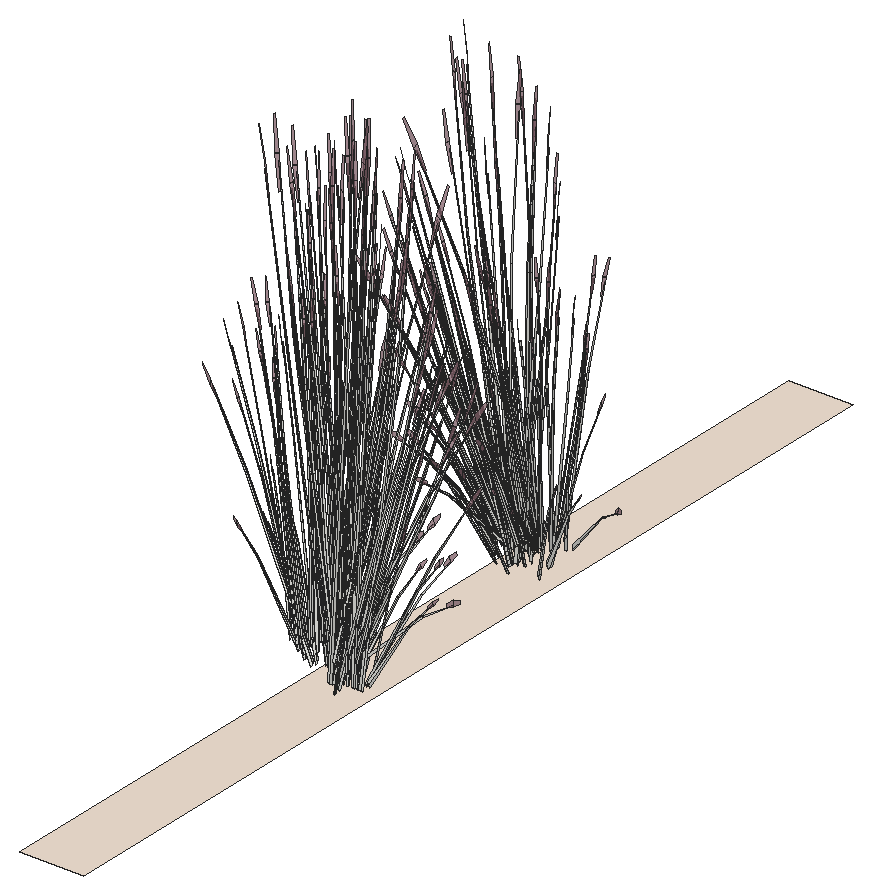
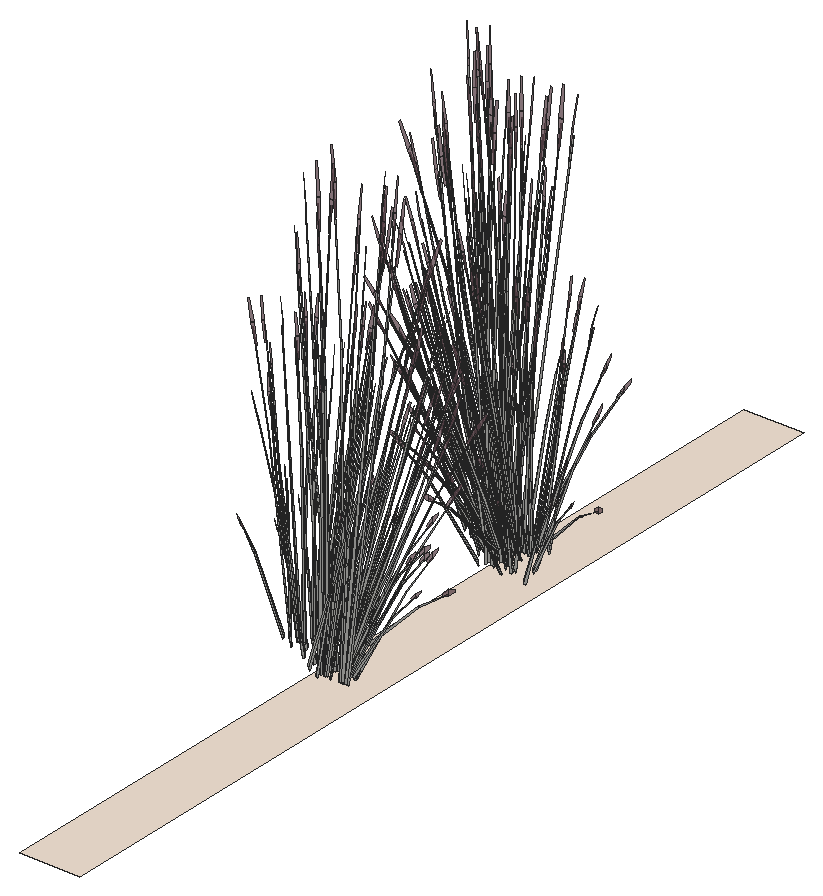
# SketchUp Ruby script. Lengths in inches.
U = 1.inch
M = Sketchup.active_model
def pt(a) = Geom::Point3d.new(a.map { |v| v * U })
def face(e, loops, mat)
  f = e.add_face(loops[0].map { |a| pt(a) })
  loops[1..].each { |l| e.add_face(l.map { |a| pt(a) }).erase! }
  f.material = f.back_material = mat if mat
  f
end
# faces: each face lists its corners as indices into pts; further lists are holes
def faces(e, pts, list, mat = nil) = list.each { |f| face(e, (f[0].is_a?(Array) ? f : [f]).map { |l| l.map { |i| pts[i] } }, mat) }
# xy, xz, yz: faces in a plane at the given z, y or x. An outline is a flat list of corners, or four numbers for a rectangle; further outlines are holes
def ring(l) = l.size == 4 ? [[l[0], l[1]], [l[2], l[1]], [l[2], l[3]], [l[0], l[3]]] : l.each_slice(2).to_a
def flat(e, list, mat, &to3) = list.each { |f| face(e, (f[0].is_a?(Array) ? f : [f]).map { |l| ring(l).map { |u, v| to3.(u, v) } }, mat) }
def xy(e, z, list, mat = nil) = flat(e, list, mat) { |x, y| [x, y, z] }
def xz(e, y, list, mat = nil) = flat(e, list, mat) { |x, z| [x, y, z] }
def yz(e, x, list, mat = nil) = flat(e, list, mat) { |y, z| [x, y, z] }
def lines(e, pts, list) = list.each { |a, b| e.add_line(pt(pts[a]), pt(pts[b])) }
# prism: a flat outline (further loops are holes) pulled along v
def prism(e, loops, v, mat = nil)
  f = face(e, loops, mat); d = Geom::Vector3d.new(v.map { |x| x * U })
  f.pushpull(f.normal.samedirection?(d) ? d.length : -d.length)
end
def box(e, o, s, mat = nil) = prism(e, [[o, [o[0] + s[0], o[1], o[2]], [o[0] + s[0], o[1] + s[1], o[2]], [o[0], o[1] + s[1], o[2]]]], [0, 0, s[2]], mat)
def at(x, y, z, deg = 0) = Geom::Transformation.translation(pt([x, y, z])) * Geom::Transformation.rotation(ORIGIN, Z_AXIS, deg.degrees)
def axes(o, x, y, z) = Geom::Transformation.new([*x, 0, *y, 0, *z, 0, *pt(o).to_a, 1])
def part(name) = M.definitions.add(name)
# library, detail: a bought-in or finely detailed component or shape, given as its bounding box
def library(name, o, s) = part(name).tap { |d| box(d.entities, o, s) }
def detail(e, o, s) = box(e.add_group.entities, o, s)
def put(e, d, t, mat = nil) = e.add_instance(d, t).tap { |i| i.material = mat if mat }
def group(e, t, mat = nil) = e.add_group.tap { |g| g.transformation = t; g.material = mat if mat }.entities
root = M.entities
M.materials.add("C01_Vanilla_Cream").color = [244, 228, 212]
M.materials.add("LightPink_Translucent").color = [144, 107, 117]
M.materials["LightPink_Translucent"].alpha = 0.75
c1 = part("blade")
p = [[2.15,0.21,22],[0,0.17,0],[0.09,0.45,0],[2.18,0.31,22],[2.29,0.31,22],[0.38,0.45,0],
  [2.48,0.24,33],[2.49,0.24,33],[2.48,0.22,33]]
faces(c1.entities,p,[[0,1,2,3],[4,5,2,3],[6,3,4,7],[8,0,3,6]])
c2 = part("seeds")
p = [[0.3,-0.1,1.38],[-0.01,-0.03,1.59],[-0.01,-0.03,0.03],[0.14,-0.07,-0.07],[0.29,-0.03,3],[0.15,0.01,3.11]]
faces(c2.entities,p,[[0,1,2,3],[1,0,4,5]],"LightPink_Translucent")
c3 = part("blade with seeds")
put(c3.entities,c1,at(0,0,0))
put(c3.entities,c2,axes([2.4,0.25,30.99],[1.5799,-0.05474,1.17369],[-0.12525,1.92788,0.29478],[-0.07173,-0.02425,1.56792]))
xy(root,198,[[354,216,360,306.76]],"C01_Vanilla_Cream")
put(root,c3,axes([359.23,246.6875,199.52],[0.13078,0.42928,-0.23233],[-0.51941,0.1219,0.23233],[0.10471,0.0495,1.0423]))
put(root,c3,axes([360.13,248.4,201.55],[0.20448,0.33592,0.04823],[-0.37288,0.16442,0.37966],[0.16437,-0.03244,0.57892]))
put(root,c3,axes([358.1875,247.65,199.79],[-0.70367,-0.1038,0.36899],[0.1432,-0.58624,0.1448],[0.10283,0.05661,1.2811]))
put(root,c3,axes([360.09,248.29,201.55],[-0.15729,0.44921,0.36002],[-0.51712,-0.15361,0.29685],[0.20336,-0.027,0.74497]))
put(root,c3,axes([357.625,249.1,199.65],[-0.18165,-0.42474,0],[0.51872,-0.14874,0],[0,0,1.15778]))
put(root,c3,axes([357.28,248.69,199.96],[-0.1074,0.43968,0.1086],[-0.52474,-0.07632,-0.3101],[-0.0955,-0.04515,0.95058]))
put(root,c3,axes([355.24,247.55,201.79],[0.46269,0.13744,0.2656],[-0.13495,0.40096,-0.3429],[-0.18628,0.03677,0.65611]))
put(root,c3,axes([358.31,249.04,199.64],[0.5845,-0.16716,-0.14398],[0.20539,0.48152,0.00006],[0.06452,-0.01848,1.30423]))
put(root,c3,axes([358.51,249.24,199.86],[0.16083,-0.48962,0.13232],[0.58854,0.13856,0.26315],[-0.10167,0.00238,1.20305]))
put(root,c3,axes([358.375,248.13,199.66],[0.38863,0.31822,0],[-0.38863,0.31822,0],[0,0,1.2695]))
put(root,c3,axes([356.17,247.53,200.51],[0.15825,-0.07127,1.32798],[0.05457,0.4976,0.10393],[-0.34278,0.06603,0.47463]))
put(root,c3,axes([359.43,247.99,199.86],[-0.43742,-0.35886,0.13232],[0.44081,-0.34807,0.26315],[-0.04831,0.07329,1.20305]))
put(root,c3,axes([358.62,247.45,199.54],[0.57914,0.08077,-0.46765],[-0.12221,0.49823,-0.12274],[0.17283,0.06037,1.03225]))
put(root,c3,axes([361.18,248.32,200.07],[-0.34399,0.08133,0.86145],[0.16192,-0.33614,0.63294],[0.18249,0.023,0.18974]))
put(root,c3,axes([357.5,249.29,199.65],[-0.56127,-0.22118,0],[0.27012,-0.45959,0],[0,0,1.2203]))
put(root,c3,axes([357.96,248.7,199.85],[-0.54364,-0.39653,-0.18894],[0.45745,-0.44527,0.41347],[-0.14639,0.04639,1.26162]))
put(root,c3,axes([356.53,249.46,199.86],[0.52105,0.24633,0.37238],[-0.31144,0.44171,0],[-0.11867,-0.0561,1.18128]))
put(root,c3,axes([358.37,247.76,200.04],[0.27012,-0.44393,0.33554],[0.56127,0.21365,-0.16149],[0,0.10233,1.07733]))
put(root,c3,axes([361.02,249.74,201.53],[-0.05034,-0.04313,1.33037],[0.11012,-0.46232,-0.12571],[0.1983,-0.02954,0.23543]))
put(root,c3,axes([354.47,247.86,201.54],[-0.09091,0.06396,1.31208],[0.00773,0.46734,-0.2075],[-0.20839,0.06078,0.10523]))
put(root,c3,axes([358.27,248.01,199.72],[0,0.56976,-0.04228],[-0.69617,0,0],[0,0.01791,1.34526]))
put(root,c3,axes([355.07,247.8,201.51],[-0.15083,0.44814,-0.38324],[-0.51712,-0.15361,-0.29685],[-0.2082,0.04109,0.7333]))
put(root,c3,axes([355.05,247.42,201.78],[0.28012,0.44611,-0.0912],[-0.49717,0.21923,-0.50621],[-0.20951,0.05886,0.76918]))
put(root,c3,axes([358.32,247.61,199.66],[0.33445,0.41351,-0.33554],[-0.50659,0.29119,0.16149],[0.10823,0.05117,1.07733]))
put(root,c3,axes([360.58,249.35,200.95],[-0.10656,-0.41414,-0.02619],[0.50364,-0.09521,-0.11874],[0.10517,0.02626,0.39164]))
put(root,c3,axes([356.23,249.72,199.78],[-0.34808,0.49367,0],[-0.58235,-0.27531,-0.38706],[-0.13264,-0.0627,1.22783]))
put(root,c3,axes([359.27,249.34,201.78],[0.02981,-0.50103,-0.0912],[0.56442,0.01369,-0.50621],[0.21738,0.0348,0.76918]))
put(root,c3,axes([359.79,248,199.86],[0,-0.49266,0.37238],[0.62289,0,0],[0,0.11221,1.18128]))
put(root,c3,axes([358.23,248.37,200.04],[0.60457,-0.03041,0.33554],[0.05467,0.50484,-0.16149],[-0.10823,0.05117,1.07733]))
put(root,c3,axes([358.6,247.86,199.96],[0.51872,-0.14368,0.1086],[0.18165,0.41027,-0.3101],[0,0.09029,0.95058]))
put(root,c3,axes([359.1875,249.15,201.79],[-0.31678,-0.30846,0.2656],[0.36171,-0.29199,-0.3429],[0.18378,0.04443,0.65611]))
put(root,c3,axes([357.6875,248.62,199.66],[-0.60457,0.03041,-0.33554],[-0.05467,-0.50484,0.16149],[-0.10823,0.05117,1.07733]))
put(root,c3,axes([360.53,248.86,199.94],[-0.13408,-0.12117,1.07251],[0.17446,-0.40083,-0.23066],[0.27128,0.0543,0.45856]))
put(root,c3,axes([358.14,249.3,199.65],[0.56127,0.22118,0],[-0.27012,0.45959,0],[0,0,1.31215]))
put(root,c3,axes([359.76,249.04,201.54],[0.11943,-0.00833,1.31208],[0.32759,-0.38275,-0.2075],[0.21244,0.05052,0.10523]))
put(root,c3,axes([358.36,249.79,199.64],[-0.34375,-0.4954,-0.03857],[0.58235,-0.27531,0.38706],[-0.1435,0.04717,1.22723]))
put(root,c3,axes([358.24,248.59,199.96],[0.41131,0.296,0.1086],[-0.34309,0.33395,-0.3101],[-0.0955,0.04515,0.95058]))
put(root,c3,axes([354.99,248.67,201.55],[-0.13808,-0.45342,0.36002],[0.54163,-0.07869,0.29685],[-0.15963,0.10664,0.74497]))
put(root,c3,axes([354.88,248.58,201.55],[-0.3822,-0.20719,0.04823],[0.22252,-0.29505,0.37966],[-0.12254,0.09539,0.57892]))
put(root,c3,axes([355.06,248.03,200.91],[0.19317,-0.10421,1.28532],[0.16263,0.48153,0.10393],[-0.30326,0.10883,0.54946]))
put(root,c3,axes([359.3,249.1,201.74],[0.55654,0.01186,-0.53284],[-0.03738,0.49951,0.0643],[0.23578,0.05271,0.75375]))
put(root,c3,axes([358.67,249.5,199.86],[0.52105,-0.24633,0.37238],[0.31144,0.44171,0],[-0.11867,0.0561,1.18128]))
put(root,c3,axes([357.93,249.11,199.72],[0.24206,0.56598,-0.04509],[-0.69162,0.19832,0],[0.00845,0.01976,1.2913]))
put(root,c3,axes([358.2,249.72,199.52],[-0.51941,-0.1219,-0.23233],[0.13078,-0.42928,0.23233],[-0.10471,0.0495,1.0423]))
put(root,c3,axes([354.45,248.85,199.94],[0.19348,0.04044,1.07251],[0.1247,0.41309,-0.23066],[-0.26282,0.07733,0.45856]))
put(root,c3,axes([355.32,248.52,201.79],[0.48462,-0.07041,0.2656],[0.12797,0.4025,-0.3429],[-0.13888,0.10811,0.65611]))
put(root,c3,axes([360.21,248.09,199.78],[0.69617,0,0],[0,0.55062,-0.38706],[0,0.12541,1.22783]))
put(root,c3,axes([353.46,248.34,201.53],[0.07105,0.01321,1.33037],[0.2198,0.43529,-0.12571],[-0.14545,0.11425,0.23543]))
put(root,c3,axes([359.93,248.37,199.65],[-0.69582,-0.00394,-0.03732],[0,-0.55062,0.37457],[-0.02187,0.12535,1.18764]))
put(root,c3,axes([358.43,247.89,200],[0.62699,0.23507,-0.21822],[-0.3019,0.49615,-0.37502],[0.0197,0.12182,1.19781]))
put(root,c3,axes([354.05,249.72,200.07],[0.23202,-0.22328,0.86145],[0.09155,0.35348,0.63294],[-0.16768,0.06329,0.18974]))
put(root,c3,axes([359.64,249.31,201.39],[0.31678,0.30846,-0.2656],[-0.36171,0.29199,0.3429],[0.18378,0.04443,0.65611]))
put(root,c3,axes([359.79,248.45,199.52],[-0.38863,0.30738,-0.23233],[-0.38863,-0.30738,0.23233],[0,0.09901,1.0423]))
put(root,c3,axes([358.11,248.48,200],[0.06488,0.56215,-0.21822],[-0.6757,0.03399,-0.37502],[-0.11898,0.07488,1.19781]))
put(root,c3,axes([359.47,249.42,201.55],[-0.02803,0.37463,0.04823],[-0.42332,-0.01027,0.37966],[0.16216,0.0392,0.57892]))
put(root,c3,axes([358.36,248.26,199.66],[-0.27012,0.44393,-0.33554],[-0.56127,-0.21365,0.16149],[0,0.10233,1.07733]))
put(root,c3,axes([354.93,248.75,201.39],[-0.48462,0.07041,-0.2656],[-0.12797,-0.4025,0.3429],[-0.13888,0.10811,0.65611]))
put(root,c3,axes([359.51,249.31,201.55],[-0.41051,0.32462,0.36002],[-0.35404,-0.34474,0.29685],[0.1926,0.05988,0.74497]))
put(root,c3,axes([354.22,249.66,202.23],[0.49129,0.13151,-0.04866],[-0.15113,0.40475,-0.22062],[-0.08035,0.06145,0.72768]))
put(root,c3,axes([357.71,248.91,199.54],[-0.375,0.3703,-0.46765],[-0.46584,-0.33578,-0.12274],[-0.15027,0.09237,1.03225]))
put(root,c3,axes([358.21,249.68,201.79],[-0.08599,-0.39682,0.2656],[0.49155,-0.10478,-0.3429],[0.13203,0.11372,0.65611]))
put(root,c3,axes([358.375,249.53,199.75],[0.697,0.16013,0.23067],[-0.17437,0.57237,-0.27369],[-0.11536,0.07164,1.23664]))
put(root,c3,axes([358.32,249.92,199.51],[-0.52105,0.24633,-0.37238],[-0.31144,-0.44171,0],[-0.11867,0.0561,1.18128]))
put(root,c3,axes([360.06,248.46,199.51],[0,0.49266,-0.37238],[-0.62289,0,0],[0,0.11221,1.18128]))
put(root,c3,axes([358.5,248.52,200.91],[-0.2068,-0.08488,1.28532],[0.42797,-0.35609,0.10393],[0.26673,0.16064,0.54946]))
put(root,c3,axes([358.54,247.4,201.36],[-0.48108,-0.25598,1.03712],[0.50798,-0.39855,0.44749],[0.15521,0.24018,1.00248]))
put(root,c3,axes([355.07,248.48,201.78],[0.515,0.27165,-0.0912],[-0.2967,0.3934,-0.50621],[-0.1455,0.13675,0.76918]))
put(root,c3,axes([359.26,249.48,200.07],[-0.31347,-0.14166,0.86145],[0.40476,-0.14393,0.63294],[0.10917,0.12192,0.18974]))
put(root,c3,axes([358.16,249.89,201.78],[0.33176,-0.4217,-0.0912],[0.48044,0.24295,-0.50621],[0.16701,0.11914,0.76918]))
put(root,c3,axes([355.76,248.36,200.91],[0.13906,-0.15138,1.28532],[0.35111,0.40859,0.10393],[-0.24082,0.18608,0.54946]))
put(root,c3,axes([355.33,248.8,201.51],[0.14302,0.44985,-0.38324],[-0.54163,0.07869,-0.29685],[-0.15522,0.12083,0.7333]))
put(root,c3,axes([355.98,249.32,201.79],[0.3767,-0.25939,0.2656],[0.3566,0.29618,-0.3429],[-0.05426,0.15048,0.65611]))
put(root,c3,axes([358.8,249.84,199.78],[0.34808,0.49367,0],[-0.58235,0.27531,-0.38706],[-0.13264,0.0627,1.22783]))
put(root,c3,axes([357.73,250.24,201.53],[0.00165,-0.05965,1.33037],[0.47711,-0.26315,-0.12571],[0.16572,0.09393,0.23543]))
put(root,c3,axes([359.35,250.01,199.12],[0.04056,-0.07113,1.32257],[0.51066,-0.20948,-0.20205],[0.15482,0.10842,0.22528]))
put(root,c3,axes([358.5,247.89,200.13],[-0.01521,-0.46386,1.05954],[0.68831,0.12024,0.44862],[-0.1628,0.25382,1.00012]))
put(root,c3,axes([358.68,248.39,199.57],[0.20414,0.45107,-0.51909],[-0.58805,0.16245,-0.13624],[0.02256,0.15274,1.1458]))
put(root,c3,axes([355.63,249.55,201.55],[-0.45752,-0.02296,0.04823],[0.01254,-0.34663,0.37966],[-0.04787,0.13278,0.57892]))
put(root,c3,axes([354.66,249.95,199.12],[0.07468,0.04922,1.32257],[0.12663,0.45605,-0.20205],[-0.16551,0.09725,0.22528]))
put(root,c3,axes([355.78,249.58,201.55],[-0.39645,-0.33614,0.36002],[0.42102,-0.2899,0.29685],[-0.07313,0.15771,0.74497]))
put(root,c3,axes([358.56,249.68,201.51],[0.54938,-0.11711,-0.38324],[0.0961,0.44351,-0.29685],[0.14756,0.1271,0.7333]))
put(root,c3,axes([357.03,249.74,201.79],[0.16784,-0.37886,0.2656],[0.48968,0.1105,-0.3429],[0.0449,0.15254,0.65611]))
put(root,c3,axes([359.3125,250.13,200],[-0.35702,-0.01545,0.78795],[0.23577,-0.32816,0.43504],[0.14104,0.11659,0.61808]))
put(root,c3,axes([358.29,250.04,201.55],[-0.25304,0.31296,0.04823],[-0.36033,-0.18221,0.37966],[0.11649,0.10034,0.57892]))
put(root,c3,axes([357.69,251.1,202.23],[0.38473,-0.28263,-0.04866],[0.35252,0.30954,-0.22062],[0.02482,0.08771,0.72768]))
put(root,c3,axes([358.39,249.95,201.55],[-0.55374,0.11306,0.36002],[-0.0961,-0.44351,0.29685],[0.13023,0.13071,0.74497]))
put(root,c3,axes([355.66,248.73,200.91],[0.10366,-0.16934,1.28532],[0.43488,0.35044,0.10393],[-0.19618,0.21841,0.54946]))
put(root,c3,axes([358.15,249.33,199.94],[0.00982,-0.16331,1.07251],[0.4695,-0.18242,-0.23066],[0.14493,0.19547,0.45856]))
put(root,c3,axes([356.88,250.09,201.55],[-0.41024,0.16744,0.04823],[-0.2008,-0.30532,0.37966],[0.03962,0.13459,0.57892]))
put(root,c3,axes([355.78,249.69,201.39],[-0.3767,0.25939,-0.2656],[-0.3566,-0.29618,0.3429],[-0.05426,0.15048,0.65611]))
put(root,c3,axes([354.48,249.61,201.54],[-0.01384,0.09749,1.31208],[0.39274,0.33916,-0.2075],[-0.10282,0.16039,0.10523]))
put(root,c3,axes([355.74,249.39,202.05],[0.61188,0.02441,-0.10123],[-0.01672,0.46217,-0.56189],[-0.0425,0.178,0.85379]))
put(root,c3,axes([356.87,249.9,201.78],[0.54481,-0.22937,-0.0912],[0.26773,0.4071,-0.50621],[0.07188,0.17155,0.76918]))
put(root,c3,axes([357.03,250.06,201.8],[-0.54859,-0.1288,0.39962],[0.18759,-0.42344,0.32951],[0.03297,0.16652,0.82692]))
put(root,c3,axes([356.02,250.69,200.07],[-0.01441,-0.29294,0.86145],[0.36003,0.20894,0.63294],[-0.07081,0.13963,0.18974]))
put(root,c3,axes([356.97,249.99,199.12],[0.0901,-0.02681,1.32257],[0.54199,0.14755,-0.20205],[0.01585,0.1663,0.22528]))
put(root,c3,axes([356.15,249.5625,201.75],[0.39855,0.33102,-0.4254],[-0.42102,0.2899,-0.32951],[-0.06064,0.16819,0.81396]))
put(root,c3,axes([355.72,250.06,200.12],[0.50577,-0.08724,0.04881],[0.11627,0.35148,-0.64728],[-0.03206,0.17792,0.5802]))
put(root,c3,axes([357.34,249.88,201.51],[0.54728,0.1235,-0.38324],[-0.18759,0.42344,-0.29685],[0.05018,0.17048,0.7333]))
put(root,c3,axes([357.65,249.01,200.91],[-0.12726,-0.15818,1.28532],[0.58807,-0.13317,0.10393],[0.13291,0.24832,0.54946]))
put(root,c3,axes([357.09,250.14,201.39],[-0.16784,0.37886,-0.2656],[-0.48968,-0.1105,0.3429],[0.0449,0.15254,0.65611]))
put(root,c3,axes([356.03,249.41,202],[-0.01449,0.45571,-0.59145],[-0.61002,-0.03061,0.07138],[-0.06438,0.19306,0.83667]))
put(root,c3,axes([354.4375,250.61,201.53],[0.06316,-0.02974,1.33037],[0.52204,0.19785,-0.12571],[-0.01227,0.16473,0.23543]))
put(root,c3,axes([356.61,249.09,200.91],[-0.01363,-0.18909,1.28532],[0.5906,0.12544,0.10393],[-0.03653,0.26947,0.54946]))
put(root,c3,axes([357.14,249.8,201.74],[0.26572,0.40059,-0.53284],[-0.54698,0.22325,0.0643],[0.06214,0.19355,0.75375]))
put(root,c3,axes([355.6,250.43,199.94],[0.17569,-0.07772,1.07251],[0.43377,0.23434,-0.23066],[-0.12911,0.20277,0.45856]))
put(root,c3,axes([356.74,250.81,201.54],[0.07057,0.07933,1.31208],[0.56952,0.03117,-0.2075],[0.05727,0.17496,0.10523]))
put(root,c3,axes([355.83,250.05,200.52],[0.01223,-0.25433,1.15759],[0.55017,0.13434,0.15997],[-0.04767,0.27105,0.54661]))
put(root,c3,axes([356.25,270.38,200.91],[0.12726,0.15818,1.28532],[-0.58807,0.13317,0.10393],[-0.13291,-0.24832,0.54946]))
put(root,c3,axes([357.22,269.33,201.54],[-0.08515,-0.06907,1.31208],[-0.56828,0.04379,-0.2075],[-0.0907,-0.16522,0.10523]))
put(root,c3,axes([358.54,270.15,199.94],[-0.15825,0.09972,1.07251],[-0.47395,-0.17454,-0.23066],[0.08785,-0.21706,0.45856]))
put(root,c3,axes([357.82,270.5,201.74],[-0.26572,-0.40059,-0.53284],[0.54698,-0.22325,0.0643],[-0.06214,-0.19355,0.75375]))
put(root,c3,axes([356.09,269.96,199.94],[-0.03371,0.16116,1.07251],[-0.49286,0.13491,-0.23066],[-0.11521,-0.20831,0.45856]))
put(root,c3,axes([357.36,269.61,199.12],[-0.09338,0.01775,1.32257],[-0.51641,-0.1998,-0.20205],[0.00867,-0.16666,0.22528]))
put(root,c3,axes([358.92,270.89,201.74],[0.01449,-0.45571,-0.53284],[0.61002,0.03061,0.0643],[0.06438,-0.19306,0.75375]))
put(root,c3,axes([359.77,270.18,201.54],[-0.00537,-0.09805,1.31208],[-0.45391,-0.28338,-0.2075],[0.07018,-0.17178,0.10523]))
put(root,c3,axes([357.87,270.16,201.39],[0.16784,-0.37886,-0.2656],[0.48968,0.1105,0.3429],[-0.0449,-0.15254,0.65611]))
put(root,c3,axes([358.24,270.66,200.91],[-0.10366,0.16934,1.28532],[-0.43488,-0.35044,0.10393],[0.19618,-0.21841,0.54946]))
put(root,c3,axes([359.65,269.82,201.53],[-0.05654,0.03763,1.33037],[-0.55396,-0.12696,-0.12571],[-0.02005,-0.16422,0.23543]))
put(root,c3,axes([357.62,270.42,201.51],[-0.54728,-0.1235,-0.38324],[0.18759,-0.42344,-0.29685],[-0.05018,-0.17048,0.7333]))
put(root,c3,axes([357.95,269.36,200.07],[0.07142,0.28728,0.86145],[-0.3962,-0.15911,0.63294],[0.04263,-0.1471,0.18974]))
put(root,c3,axes([358.8,270.74,201.51],[-0.39855,-0.33102,-0.38324],[0.42102,-0.2899,-0.29685],[0.06064,-0.16819,0.7333]))
put(root,c3,axes([356.64,269.1,201.53],[-0.01039,0.05905,1.33037],[-0.51226,0.21431,-0.12571],[-0.15074,-0.10955,0.23543]))
put(root,c3,axes([356.52,270.15,201.82],[0.62019,-0.12663,0.40322],[0.10763,0.49673,0.33247],[-0.14586,-0.1464,0.83437]))
put(root,c3,axes([357.93,270.24,201.55],[0.54859,0.1288,0.36002],[-0.18759,0.42344,0.29685],[-0.03297,-0.16652,0.74497]))
put(root,c3,axes([358.08,270.4,201.78],[-0.54481,0.22937,-0.0912],[-0.26773,-0.4071,-0.50621],[-0.07188,-0.17155,0.76918]))
put(root,c3,axes([359.22,270.91,201.78],[-0.61188,-0.02441,-0.0912],[0.01672,-0.46217,-0.50621],[0.0425,-0.178,0.76918]))
put(root,c3,axes([359.17,270.61,201.39],[0.3767,-0.25939,-0.2656],[0.3566,0.29618,0.3429],[0.05426,-0.15048,0.65611]))
put(root,c3,axes([355.92,269.7,200.07],[0.29042,0.17147,0.86145],[-0.42295,0.10307,0.63294],[-0.0905,-0.13178,0.18974]))
put(root,c3,axes([358.07,270.21,201.55],[0.41024,-0.16744,0.04823],[0.2008,0.30532,0.37966],[-0.03962,-0.13459,0.57892]))
put(root,c3,axes([356.62,270.61,201.74],[-0.47473,-0.23813,-0.53284],[0.33738,-0.41728,0.0643],[-0.172,-0.14218,0.75375]))
put(root,c3,axes([356.45,270.29,201.39],[-0.08599,-0.39682,-0.2656],[0.49155,-0.10478,0.3429],[-0.13203,-0.11372,0.65611]))
put(root,c3,axes([356.67,270.26,201.55],[0.25304,-0.31296,0.04823],[0.36033,0.18221,0.37966],[-0.11649,-0.10034,0.57892]))
put(root,c3,axes([355.6875,270.22,199.12],[-0.05393,0.0649,1.32257],[-0.545,0.13993,-0.20205],[-0.13166,-0.12729,0.22528]))
put(root,c3,axes([356.59,272,199.57],[-0.22864,-0.5052,-0.52377],[0.65862,-0.18195,-0.13747],[-0.02527,-0.17107,1.15612]))
put(root,c3,axes([355.4,270.87,200.91],[0.2068,0.08488,1.28532],[-0.42797,0.35609,0.10393],[-0.26673,-0.16064,0.54946]))
put(root,c3,axes([359.64,270.46,199.12],[-0.08333,-0.03881,1.32257],[-0.21404,-0.4336,-0.20205],[0.14439,-0.11767,0.22528]))
put(root,c3,axes([357.92,270.55,201.79],[-0.16784,0.37886,0.2656],[-0.48968,-0.1105,-0.3429],[-0.0449,-0.15254,0.65611]))
put(root,c3,axes([356.4,270.62,201.51],[-0.54938,0.11711,-0.38324],[-0.0961,-0.44351,-0.29685],[-0.14756,-0.1271,0.7333]))
put(root,c3,axes([359.17,270.71,201.55],[0.39645,0.33614,0.36002],[-0.42102,0.2899,0.29685],[0.07313,-0.15771,0.74497]))
put(root,c3,axes([356.78,270.23,202.07],[-0.37157,0.4723,-0.10215],[-0.5381,-0.2721,-0.56695],[-0.18705,-0.13344,0.86148]))
put(root,c3,axes([359.32,270.75,201.55],[0.45752,0.02296,0.04823],[-0.01254,0.34663,0.37966],[0.04787,-0.13278,0.57892]))
put(root,c3,axes([358.98,270.98,201.79],[-0.3767,0.25939,0.2656],[-0.3566,-0.29618,-0.3429],[0.05426,-0.15048,0.65611]))
put(root,c3,axes([359.64,271.68,201.74],[0.29081,-0.38873,-0.53284],[0.5096,0.27626,0.0643],[0.17364,-0.14084,0.75375]))
put(root,c3,axes([356.5,270.55,199.78],[-0.34808,-0.49367,0],[0.58235,-0.27531,-0.38706],[0.13264,-0.0627,1.22783]))
put(root,c3,axes([359.625,271.5,201.51],[-0.14302,-0.44985,-0.38324],[0.54163,-0.07869,-0.29685],[0.15522,-0.12083,0.7333]))
put(root,c3,axes([357.26,269.95,199.6],[-0.38473,0.28263,-0.02919],[-0.35252,-0.30954,-0.13237],[-0.02482,-0.08771,0.43661]))
put(root,c3,axes([355.36,270.09,201.54],[-0.11979,-0.00348,1.31208],[-0.38137,0.34775,-0.2075],[-0.20349,-0.07106,0.10523]))
put(root,c3,axes([359.88,271.82,201.78],[-0.515,-0.27165,-0.0912],[0.2967,-0.3934,-0.50621],[0.1455,-0.13675,0.76918]))
put(root,c3,axes([357.75,273.3,200.49],[0.48111,0.19866,1.13446],[-0.47133,0.42798,0.44862],[-0.21112,-0.25366,0.95105]))
put(root,c3,axes([356.75,270.62,201.79],[0.08599,0.39682,0.2656],[-0.49155,0.10478,-0.3429],[-0.13203,-0.11372,0.65611]))
put(root,c3,axes([355.24,271.93,199.51],[0,-0.49266,-0.37238],[0.62289,0,0],[0,-0.11221,1.18128]))
put(root,c3,axes([356.97,270.47,199.51],[0.52105,-0.24633,-0.37238],[0.31144,0.44171,0],[0.11867,-0.0561,1.18128]))
put(root,c3,axes([360.0625,271.32,199.94],[-0.19889,-0.01459,1.07251],[-0.20376,-0.39145,-0.23066],[0.24434,-0.11074,0.45856]))
put(root,c3,axes([355.27,270.875,201.82],[0.45978,-0.36358,0.40322],[0.39653,0.38611,0.33247],[-0.21571,-0.06707,0.83437]))
put(root,c3,axes([361.15,271.7,201.53],[-0.07272,-0.00374,1.33037],[-0.30197,-0.40092,-0.12571],[0.12127,-0.13182,0.23543]))
put(root,c3,axes([357.59,271.48,199.54],[0.375,-0.3703,-0.46765],[0.46584,0.33578,-0.12274],[0.15027,-0.09237,1.03225]))
put(root,c3,axes([360.29,270.6,200.07],[-0.18544,0.25079,0.86145],[-0.15939,-0.33694,0.63294],[0.15316,-0.08443,0.18974]))
put(root,c3,axes([360.03,271.55,201.39],[0.48462,-0.07041,-0.2656],[0.12797,0.4025,0.3429],[0.13888,-0.10811,0.65611]))
put(root,c3,axes([355.48,270.875,201.55],[0.02803,-0.37463,0.04823],[0.42332,0.01027,0.37966],[-0.16216,-0.0392,0.57892]))
put(root,c3,axes([356.93,272.13,199.66],[0.27012,-0.44393,-0.33554],[0.56127,0.21365,0.16149],[0,-0.10233,1.07733]))
put(root,c3,axes([355.32,270.99,201.39],[-0.31678,-0.30846,-0.2656],[0.36171,-0.29199,0.3429],[-0.18378,-0.04443,0.65611]))
put(root,c3,axes([357.18,271.91,200],[-0.06488,-0.56215,-0.21822],[0.6757,-0.03399,-0.37502],[0.11898,-0.07488,1.19781]))
put(root,c3,axes([355.51,271.94,199.52],[0.38863,-0.30738,-0.23233],[0.38863,0.30738,0.23233],[0,-0.09901,1.0423]))
put(root,c3,axes([355.35,270.47,199.6],[-0.1606,0.40228,-0.02919],[-0.4943,-0.12375,-0.13237],[-0.07505,-0.0658,0.43661]))
put(root,c3,axes([359.63,271.78,201.79],[-0.48462,0.07041,0.2656],[-0.12797,-0.4025,-0.3429],[0.13888,-0.10811,0.65611]))
put(root,c3,axes([356.87,272.5,200],[-0.62699,-0.23507,-0.21822],[0.3019,-0.49615,-0.37502],[-0.0197,-0.12182,1.19781]))
put(root,c3,axes([355.08,272.3,199.78],[-0.69617,0,0],[0,-0.55062,-0.38706],[0,-0.12541,1.22783]))
put(root,c3,axes([355.2,271.32,199.94],[0.1087,0.13716,1.07251],[-0.25048,0.37284,-0.23066],[-0.25719,-0.08912,0.45856]))
put(root,c3,axes([357.09,270.67,199.52],[0.51941,0.1219,-0.23233],[-0.13078,0.42928,0.23233],[0.10471,-0.0495,1.0423]))
put(root,c3,axes([355.65,271.2,201.74],[-0.55654,-0.01186,-0.53284],[0.03738,-0.49951,0.0643],[-0.23578,-0.05271,0.75375]))
put(root,c3,axes([360.07,271.72,201.55],[0.3822,0.20719,0.04823],[-0.22252,0.29505,0.37966],[0.12254,-0.09539,0.57892]))
put(root,c3,axes([359.96,271.63,201.55],[0.13808,0.45342,0.36002],[-0.54163,0.07869,0.29685],[0.15963,-0.10664,0.74497]))
put(root,c3,axes([361.42,272.18,201.54],[0.07726,-0.07504,1.31208],[-0.09888,-0.46032,-0.2075],[0.19384,-0.08728,0.10523]))
put(root,c3,axes([355.625,272.16,199.75],[-0.51786,0.4142,0.23067],[-0.51817,-0.40984,-0.27369],[-0.01808,-0.11762,1.23664]))
put(root,c3,axes([354.9,270.38,201.53],[0.04127,0.04917,1.33037],[-0.19898,0.44196,-0.12571],[-0.20151,0.0032,0.23543]))
put(root,c3,axes([357.27,272.35,199.82],[0.6273,0.23878,0.18048],[-0.3019,0.49615,0.37502],[0,-0.11437,1.20407]))
put(root,c3,axes([357.03,273.02,199.83],[0.14756,-0.58378,-0.17572],[0.69966,0.10176,0.38453],[-0.12225,-0.08062,1.1733]))
put(root,c3,axes([355.47,271.3,201.51],[-0.40426,0.32635,-0.38324],[-0.35404,-0.34474,-0.29685],[-0.2054,-0.04965,0.7333]))
put(root,c3,axes([355.77,271.15,201.79],[0.31678,0.30846,0.2656],[-0.36171,0.29199,-0.3429],[-0.18378,-0.04443,0.65611]))
put(root,c3,axes([354.56,271.73,200.07],[0.35544,-0.03525,0.86145],[-0.22547,0.31061,0.63294],[-0.17565,-0.04659,0.18974]))
put(root,c3,axes([357.07,272.02,200.04],[-0.60457,0.03041,0.33554],[-0.05467,-0.50484,-0.16149],[0.10823,-0.05117,1.07733]))
put(root,c3,axes([355.68,270.96,201.78],[-0.02981,0.50103,-0.0912],[-0.56442,-0.01369,-0.50621],[-0.21738,-0.0348,0.76918]))
put(root,c3,axes([355.51,272.39,199.86],[0,0.49266,0.37238],[-0.62289,0,0],[0,-0.11221,1.18128]))
put(root,c3,axes([359.9,272.88,201.78],[-0.28012,-0.44611,-0.0912],[0.49717,-0.21923,-0.50621],[0.20951,-0.05886,0.76918]))
